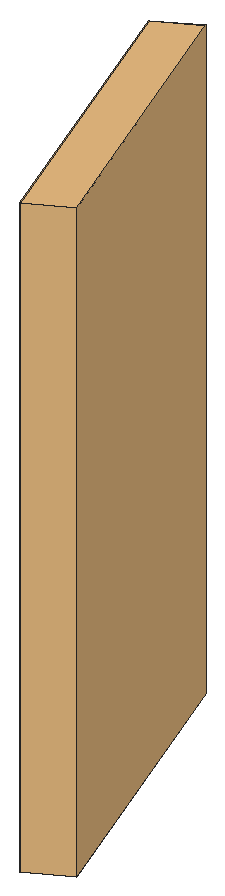
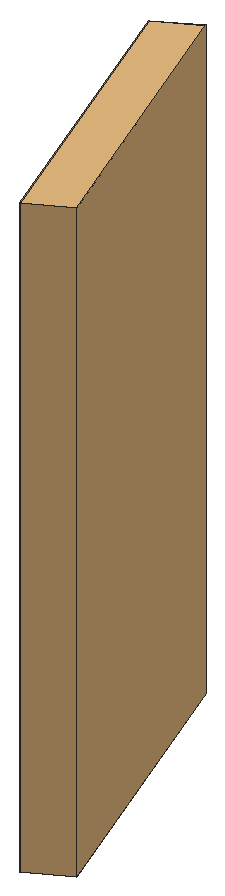
# SketchUp Ruby script. Lengths in inches.
U = 1.inch
M = Sketchup.active_model
def pt(a) = Geom::Point3d.new(a.map { |v| v * U })
def face(e, loops, mat)
  f = e.add_face(loops[0].map { |a| pt(a) })
  loops[1..].each { |l| e.add_face(l.map { |a| pt(a) }).erase! }
  f.material = f.back_material = mat if mat
  f
end
# faces: each face lists its corners as indices into pts; further lists are holes
def faces(e, pts, list, mat = nil) = list.each { |f| face(e, (f[0].is_a?(Array) ? f : [f]).map { |l| l.map { |i| pts[i] } }, mat) }
# xy, xz, yz: faces in a plane at the given z, y or x. An outline is a flat list of corners, or four numbers for a rectangle; further outlines are holes
def ring(l) = l.size == 4 ? [[l[0], l[1]], [l[2], l[1]], [l[2], l[3]], [l[0], l[3]]] : l.each_slice(2).to_a
def flat(e, list, mat, &to3) = list.each { |f| face(e, (f[0].is_a?(Array) ? f : [f]).map { |l| ring(l).map { |u, v| to3.(u, v) } }, mat) }
def xy(e, z, list, mat = nil) = flat(e, list, mat) { |x, y| [x, y, z] }
def xz(e, y, list, mat = nil) = flat(e, list, mat) { |x, z| [x, y, z] }
def yz(e, x, list, mat = nil) = flat(e, list, mat) { |y, z| [x, y, z] }
def lines(e, pts, list) = list.each { |a, b| e.add_line(pt(pts[a]), pt(pts[b])) }
# prism: a flat outline (further loops are holes) pulled along v
def prism(e, loops, v, mat = nil)
  f = face(e, loops, mat); d = Geom::Vector3d.new(v.map { |x| x * U })
  f.pushpull(f.normal.samedirection?(d) ? d.length : -d.length)
end
def box(e, o, s, mat = nil) = prism(e, [[o, [o[0] + s[0], o[1], o[2]], [o[0] + s[0], o[1] + s[1], o[2]], [o[0], o[1] + s[1], o[2]]]], [0, 0, s[2]], mat)
def at(x, y, z, deg = 0) = Geom::Transformation.translation(pt([x, y, z])) * Geom::Transformation.rotation(ORIGIN, Z_AXIS, deg.degrees)
def axes(o, x, y, z) = Geom::Transformation.new([*x, 0, *y, 0, *z, 0, *pt(o).to_a, 1])
def part(name) = M.definitions.add(name)
# library, detail: a bought-in or finely detailed component or shape, given as its bounding box
def library(name, o, s) = part(name).tap { |d| box(d.entities, o, s) }
def detail(e, o, s) = box(e.add_group.entities, o, s)
def put(e, d, t, mat = nil) = e.add_instance(d, t).tap { |i| i.material = mat if mat }
def group(e, t, mat = nil) = e.add_group.tap { |g| g.transformation = t; g.material = mat if mat }.entities
root = M.entities
c1 = library("sm2 st v2 Component\#1",[0,0,0],[29.46,4.93,43.46])
put(root,c1,axes([78.91,83.01,57.27],[-0.16628,0.46803,0],[-0.37701,-0.20642,0],[0,0,0.6557]))
